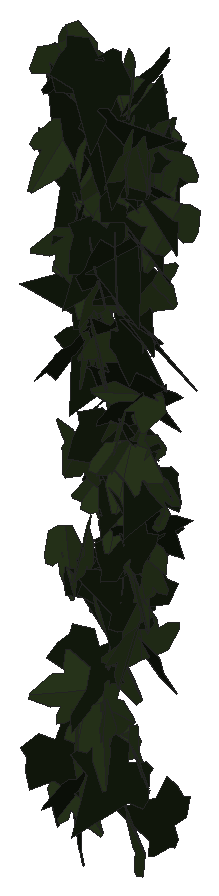
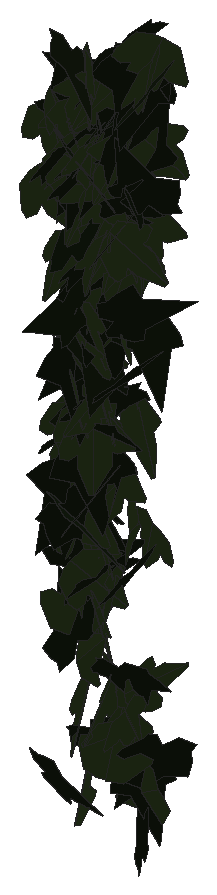
# SketchUp Ruby script. Lengths in inches.
U = 1.inch
M = Sketchup.active_model
def pt(a) = Geom::Point3d.new(a.map { |v| v * U })
def face(e, loops, mat)
  f = e.add_face(loops[0].map { |a| pt(a) })
  loops[1..].each { |l| e.add_face(l.map { |a| pt(a) }).erase! }
  f.material = f.back_material = mat if mat
  f
end
# faces: each face lists its corners as indices into pts; further lists are holes
def faces(e, pts, list, mat = nil) = list.each { |f| face(e, (f[0].is_a?(Array) ? f : [f]).map { |l| l.map { |i| pts[i] } }, mat) }
# xy, xz, yz: faces in a plane at the given z, y or x. An outline is a flat list of corners, or four numbers for a rectangle; further outlines are holes
def ring(l) = l.size == 4 ? [[l[0], l[1]], [l[2], l[1]], [l[2], l[3]], [l[0], l[3]]] : l.each_slice(2).to_a
def flat(e, list, mat, &to3) = list.each { |f| face(e, (f[0].is_a?(Array) ? f : [f]).map { |l| ring(l).map { |u, v| to3.(u, v) } }, mat) }
def xy(e, z, list, mat = nil) = flat(e, list, mat) { |x, y| [x, y, z] }
def xz(e, y, list, mat = nil) = flat(e, list, mat) { |x, z| [x, y, z] }
def yz(e, x, list, mat = nil) = flat(e, list, mat) { |y, z| [x, y, z] }
def lines(e, pts, list) = list.each { |a, b| e.add_line(pt(pts[a]), pt(pts[b])) }
# prism: a flat outline (further loops are holes) pulled along v
def prism(e, loops, v, mat = nil)
  f = face(e, loops, mat); d = Geom::Vector3d.new(v.map { |x| x * U })
  f.pushpull(f.normal.samedirection?(d) ? d.length : -d.length)
end
def box(e, o, s, mat = nil) = prism(e, [[o, [o[0] + s[0], o[1], o[2]], [o[0] + s[0], o[1] + s[1], o[2]], [o[0], o[1] + s[1], o[2]]]], [0, 0, s[2]], mat)
def at(x, y, z, deg = 0) = Geom::Transformation.translation(pt([x, y, z])) * Geom::Transformation.rotation(ORIGIN, Z_AXIS, deg.degrees)
def axes(o, x, y, z) = Geom::Transformation.new([*x, 0, *y, 0, *z, 0, *pt(o).to_a, 1])
def part(name) = M.definitions.add(name)
# library, detail: a bought-in or finely detailed component or shape, given as its bounding box
def library(name, o, s) = part(name).tap { |d| box(d.entities, o, s) }
def detail(e, o, s) = box(e.add_group.entities, o, s)
def put(e, d, t, mat = nil) = e.add_instance(d, t).tap { |i| i.material = mat if mat }
def group(e, t, mat = nil) = e.add_group.tap { |g| g.transformation = t; g.material = mat if mat }.entities
root = M.entities
M.materials.add("efeu1").color = [18, 25, 13]
M.materials.add("efeu2").color = [43, 57, 29]
c1 = part("ivyleaf_9")
p = [[1.54,2.16,1.25],[1.36,2.04,1.19],[-0.21,0.99,0.68],[-0.71,1.11,0.82],[-0.85,0.86,0.67],[-0.8,0.17,0.21],
  [-0.9,-0.01,0.1],[-0.67,-0.16,-0.02],[-0.08,-0.08,-0.05],[-0.03,-0.6,-0.4],[0.65,-0.88,-0.66],[0.83,-0.6,-0.49],
  [1.29,-0.42,-0.43],[1.8125,-0.07,-0.26],[1.21,0.44,0.15]]
faces(c1.entities,p,[[0,1,2,3,4,5,6,7,8,9,10,11,12,13,14]],"efeu1")
c2 = part("ivyleaf_10")
p = [[0,0.5,-0.03],[-0.0625,2.02,-0.43],[-0.19,2.01,-0.46],[-0.54,1.05,-0.29],[-0.52,0.625,-0.18],[-0.83,0.76,-0.28],
  [-1.16,0.64,-0.33],[-1.15,0.33,-0.24],[-0.77,-0.39,0.02],[-0.3,-0.51,0.16],[0.04,-0.48,0.23],[-0.02,2.01,-0.4375],
  [-0.06,2.01,-0.43],[0.04,-0.49,0.23],[0.67,-0.49,0.14],[1.38,0.36,-0.2],[1.375,0.51,-0.24],[0.81,0.65,-0.19],
  [0.62,0.59,-0.15],[0.6,1.09,-0.28],[0.5,1.23,-0.31]]
faces(c2.entities,p,[[0,1,2,3,4,5,6,7,8,9,10],[11,12,0,13,14,15,16,17,18,19,20]],"efeu2")
put(root,c1,axes([505.9,134.97,202.1],[-0.48741,0.05038,0.54087],[0.53842,-0.16422,0.46647],[0.16894,0.66872,0.0738]))
put(root,c2,axes([506.2,134.38,203.4],[0.33617,0.52917,-0.48557],[-0.31185,-0.37012,-0.63647],[-0.69544,0.42176,0.05069]))
put(root,c2,axes([505.99,134.85,205.88],[-0.15088,0.81193,-0.1575],[0.02758,-0.15507,-0.82583],[-0.82661,-0.15338,0.00119]))
put(root,c1,axes([506.57,135.38,198.56],[-0.26804,-0.09847,0.66727],[-0.6448,-0.23495,-0.27769],[0.27513,-0.64656,-0.00072]))
put(root,c1,axes([505.92,134.4,185.77],[-0.02694,-0.41849,-0.61943],[0.0465,0.59407,-0.43597],[0.78479,-0.04957,0.00457]))
put(root,c1,axes([505.94,135.15,183.02],[0.03534,-0.05301,0.72791],[0.1299,-0.68989,-0.06019],[0.74686,0.1225,-0.02398]))
put(root,c2,axes([506.81,134.96,200.54],[-0.36293,-0.14169,0.65201],[-0.60869,-0.27512,-0.37885],[0.33369,-0.65595,0.01806]))
put(root,c2,axes([506.47,134.6,187.4],[-0.10798,0.2032,0.71797],[-0.06576,-0.69688,0.20416],[0.77443,-0.03084,0.11744]))
put(root,c1,axes([505.91,134.95,205.33],[0.46062,-0.69476,-0.084],[0.0295,0.11975,-0.82867],[0.6992,0.45264,0.0903]))
put(root,c2,axes([506.36,135.26,186.92],[0.0782,0.58891,-0.37757],[-0.09629,-0.35405,-0.61577],[-0.74094,0.10817,0.04017]))
put(root,c2,axes([506.34,134.14,205.99],[-0.6972,-0.29211,-0.29478],[0.28746,0.09911,-0.73668],[0.33257,-0.69804,0.01877]))
put(root,c1,axes([506.6875,134.23,185],[-0.10898,0.67608,-0.20617],[0.0546,-0.1928,-0.71058],[-0.75894,-0.11095,-0.02152]))
put(root,c1,axes([506.54,135.14,202.08],[-0.43183,-0.55961,0.15094],[-0.09356,-0.11648,-0.71528],[0.61732,-0.40911,-0.00282]))
put(root,c1,axes([506.75,134.56,203.08],[0.50705,-0.04173,0.6532],[-0.6402,0.23427,0.47702],[-0.22869,-0.74835,0.11291]))
put(root,c1,axes([506.52,135.29,188.28],[-0.62142,-0.36737,-0.26252],[0.27785,0.06288,-0.70506],[0.39311,-0.62517,0.08335]))
put(root,c1,axes([506.85,133.81,197.85],[-0.14356,0.79952,-0.03224],[0.00115,-0.03125,-0.84291],[-0.86413,-0.13287,0.00423]))
put(root,c1,axes([506.61,134.27,205.44],[0.38487,0.63053,-0.04593],[-0.0249,-0.0377,-0.75323],[-0.68218,0.3571,0.00158]))
put(root,c1,axes([506.45,135.54,196.82],[-0.23751,-0.66097,0.36817],[0.03415,-0.39486,-0.68685],[0.75582,-0.18986,0.14672]))
put(root,c2,axes([506.74,134.18,200.81],[-0.5053,-0.64853,-0.00396],[0.00139,0.00376,-0.83167],[0.70043,-0.46787,-0.0012]))
put(root,c2,axes([506.03,134.62,184.59],[0.3965,-0.01317,0.74077],[0.74088,0.00762,-0.39643],[-0.00051,0.84017,0.01521]))
put(root,c2,axes([507.08,133.88,194.84],[-0.59609,0.10057,0.49608],[-0.50667,0.08625,-0.58346],[-0.14308,-0.72438,-0.0006]))
put(root,c2,axes([506.35,134.14,191.88],[0.63807,-0.18963,0.34261],[0.35843,-0.0395,-0.64265],[0.20015,0.67529,0.05862]))
put(root,c2,axes([506.85,135.38,185.4],[-0.62781,-0.39783,-0.1863],[-0.15963,-0.09612,0.74323],[-0.40925,0.64777,-0.00412]))
put(root,c2,axes([506.74,135.08,186.35],[0.49996,0.50856,-0.14226],[-0.09978,-0.10088,-0.71521],[-0.55995,0.47206,0.00042]))
put(root,c1,axes([506.64,135.43,203.98],[-0.05797,0.05272,-0.73545],[0.56163,-0.47922,-0.0782],[-0.52067,-0.52279,-0.00247]))
put(root,c1,axes([506.61,134.42,201.55],[-0.08415,0.57535,0.55617],[0.04479,-0.53364,0.60338],[0.84716,0.08536,0.02334]))
put(root,c1,axes([506.54,134.9,190.93],[0.28868,-0.7047,-0.12037],[-0.03109,0.11731,-0.76138],[0.71423,0.28994,0.01551]))
put(root,c1,axes([506.56,135.25,201.17],[0.39928,-0.70619,-0.07102],[-0.01722,0.07183,-0.811],[0.70954,0.39914,0.02029]))
put(root,c2,axes([506.85,134.5,191.96],[-0.07688,0.20886,-0.70763],[0.12741,-0.67089,-0.22701],[-0.75806,-0.13394,0.03361]))
put(root,c2,axes([506.93,134.47,200.11],[0.8266,0.09302,0.0051],[0.00501,0.00248,-0.80184],[-0.10048,0.76538,0.00198]))
put(root,c2,axes([506.86,134.67,198.08],[0.28754,-0.5142,0.53683],[0.34895,-0.40924,-0.5973],[0.70527,0.41212,0.07667]))
put(root,c2,axes([506.96,134.61,203.16],[0.11167,0.65461,0.43041],[0.02152,0.41514,-0.68808],[-0.83614,0.09811,0.03977]))
put(root,c2,axes([507.21,134.53,190.43],[-0.2462,0.47178,0.4209],[-0.20846,0.35603,-0.54471],[-0.63813,-0.29833,0.01555]))
put(root,c2,axes([507.23,134.26,199.54],[-0.7868,0.29407,-0.09976],[0.09346,-0.04187,-0.81703],[-0.32072,-0.73361,0.00664]))
put(root,c2,axes([507.66,135.45,190.82],[-0.3494,-0.35385,0.57863],[-0.29236,-0.49382,-0.49033],[0.64933,-0.41274,0.09058]))
put(root,c2,axes([507.41,134.65,193.42],[-0.78212,-0.20437,-0.07107],[0.06891,0.02548,-0.78253],[0.22229,-0.72696,-0.00745]))
put(root,c2,axes([507.39,134.62,187.12],[0.22352,-0.47181,-0.62714],[0.06767,0.66124,-0.47335],[0.78188,0.07766,0.22025]))
put(root,c2,axes([507.2,134.45,200.51],[0.3411,0.60844,0.42613],[0.1273,0.41409,-0.69315],[-0.73183,0.35562,0.07804]))
put(root,c1,axes([507.23,134.39,205.99],[-0.07291,-0.83658,0.02971],[0.00071,-0.02989,-0.83975],[0.83711,-0.07284,0.0033]))
put(root,c2,axes([507.93,135.03,192.15],[-0.57202,0.2865,-0.47924],[-0.4593,0.18076,0.62523],[0.36396,0.67838,0.0358]))
put(root,c2,axes([507.49,135.11,189.86],[0.60838,-0.5967,0.00898],[0.00677,-0.00591,-0.85216],[0.59673,0.60842,0.00052]))
put(root,c1,axes([507.7,134.875,194.05],[0.34677,0.50768,-0.38385],[-0.20514,-0.31654,-0.62468],[-0.64609,0.37299,-0.00768]))
put(root,c2,axes([507.66,135.03,194.66],[-0.54907,-0.5484,0.00044],[0.00538,-0.00519,-0.77768],[0.59224,-0.50837,0.00747]))
put(root,c1,axes([507.37,135.2,190.65],[-0.08634,-0.75429,-0.01122],[-0.00292,0.01162,-0.7592],[0.75437,-0.08629,-0.00422]))
put(root,c1,axes([507.8,134.54,200.9],[-0.74349,-0.30747,0.00273],[-0.00234,-0.00158,-0.78412],[0.33208,-0.68842,0.00058]))
put(root,c2,axes([507.52,134.96,200.24],[-0.14291,0.68465,0.09871],[-0.034,0.09057,-0.72507],[-0.74572,-0.13533,0.01414]))
put(root,c2,axes([507.12,134.32,198.13],[0.29318,-0.3648,0.60841],[0.61302,-0.2386,-0.42867],[0.42263,0.59916,0.19972]))
put(root,c2,axes([507.99,134.8125,201.24],[0.16644,0.31389,0.63151],[-0.49349,-0.41564,0.34406],[0.54905,-0.46873,0.11781]))
put(root,c2,axes([507.49,134,200.86],[-0.28951,0.64386,-0.16028],[0.0694,-0.14018,-0.72531],[-0.71164,-0.27561,-0.00553]))
put(root,c1,axes([507.82,134.39,196.67],[0.08879,0.62516,0.36414],[-0.07213,0.35759,-0.64769],[-0.77049,0.03856,0.1026]))
put(root,c2,axes([507.48,134.0625,202.32],[0.06736,-0.29867,0.68359],[0.06153,0.65973,0.30615],[-0.7773,0.02634,0.08348]))
put(root,c2,axes([507.61,135.16,203.12],[0.07754,0.66937,-0.09632],[-0.02797,-0.09034,-0.69994],[-0.72927,0.07464,0.0166]))
put(root,c2,axes([508.07,134.82,187.9],[-0.39226,0.30403,-0.44186],[-0.36805,0.25434,0.49226],[0.42767,0.49773,0.01835]))
put(root,c2,axes([507.78,133.73,199.93],[-0.00169,-0.56015,-0.53529],[0.02763,0.51437,-0.58226],[0.8211,-0.01846,0.0185]))
put(root,c2,axes([507.67,134.63,195.62],[-0.09451,-0.27106,-0.735],[0.18417,0.68609,-0.29563],[0.79647,-0.19081,-0.01886]))
put(root,c2,axes([507.83,134.49,195.88],[0.50129,-0.58628,-0.21726],[-0.13097,0.17042,-0.77761],[0.65929,0.47963,0.01072]))
put(root,c2,axes([507.54,134.2,201.5],[-0.2278,-0.30885,-0.61673],[0.38163,0.4764,-0.38876],[0.61303,-0.41134,0.01283]))
put(root,c2,axes([507.49,134.95,191.48],[0.52123,-0.36531,0.33957],[0.31481,-0.15431,-0.62764],[0.42533,0.56189,0.04841]))
put(root,c1,axes([507.94,134.64,185.73],[-0.66676,-0.40237,0.01917],[-0.01624,-0.01018,-0.77877],[0.4025,-0.66696,0.00032]))
put(root,c2,axes([507.64,134.97,201.73],[-0.71869,-0.24262,-0.27889],[0.28265,0.06446,-0.7361],[0.26953,-0.71456,0.02829]))
put(root,c2,axes([507.76,134.95,191.85],[0.72959,-0.17745,-0.13262],[-0.08391,0.20108,-0.73069],[0.20502,0.71377,0.17287]))
put(root,c2,axes([507.79,134.34,198.17],[-0.41122,-0.54336,-0.1912],[0.1156,0.14949,-0.69003],[0.60863,-0.39552,0.00188]))
put(root,c2,axes([507.38,134.25,186.98],[0.65246,-0.25281,0.5036],[0.47256,-0.17419,-0.69969],[0.30694,0.80558,0.00674]))
put(root,c1,axes([508.375,134.98,192.12],[-0.45582,0.53306,0.31299],[-0.32523,0.13746,-0.69242],[-0.57559,-0.49981,0.14338]))
put(root,c2,axes([507.79,135.04,205.5],[0.52207,-0.6319,-0.15656],[0.03436,0.22715,-0.80224],[0.6501,0.49545,0.16813]))
put(root,c2,axes([508.02,134.86,198],[0.51558,-0.35857,-0.36785],[-0.30687,0.21066,-0.62093],[0.44914,0.55555,-0.00197]))
put(root,c1,axes([507.8125,134.26,198.52],[0.54701,0.42102,-0.21384],[-0.169,-0.13342,-0.68497],[-0.47698,0.53011,-0.00255]))
put(root,c1,axes([507.49,135.32,192.89],[0.20655,-0.75847,0.16522],[0.03911,-0.16058,-0.78608],[0.77527,0.21018,-0.00436]))
put(root,c1,axes([507.91,134.86,194.57],[-0.64244,-0.39994,-0.2115],[0.18233,0.11337,-0.74547],[0.44896,-0.61835,0.00012]))
put(root,c1,axes([508.15,135.4,192.55],[0.01162,0.16304,-0.67841],[-0.11569,-0.64365,-0.16915],[-0.7169,0.10652,0.0163]))
put(root,c1,axes([507.65,134.02,203.79],[0.50127,-0.44874,-0.41976],[-0.27302,0.31781,-0.6698],[0.59191,0.52662,0.04653]))
put(root,c2,axes([507.85,134.54,193.5625],[0.70397,0.3595,-0.09635],[-0.09813,-0.02701,-0.77389],[-0.38875,0.65782,0.02087]))
put(root,c1,axes([508.41,134.96,202.72],[-0.46894,0.44729,0.27331],[-0.20799,0.17923,-0.64819],[-0.52024,-0.47484,0.01279]))
put(root,c2,axes([507.79,134.52,200.68],[-0.22018,0.53236,-0.40274],[0.10654,-0.37611,-0.59174],[-0.70294,-0.22375,0.03646]))
put(root,c2,axes([507.99,134.7,201.125],[-0.01278,-0.2543,-0.6565],[0.02216,0.63092,-0.26474],[0.73466,-0.02345,-0.00344]))
put(root,c1,axes([507.67,134.58,195.45],[-0.10009,-0.79739,-0.26224],[0.09332,0.25189,-0.80153],[0.8342,-0.12385,0.0582]))
put(root,c1,axes([508.47,134.85,190.46],[-0.12991,0.028,0.74052],[-0.76459,-0.08688,-0.12083],[0.08759,-0.71688,0.04357]))
put(root,c2,axes([507.55,134.64,204.45],[0.5058,0.31332,0.47004],[0.39415,0.26701,-0.58581],[-0.4443,0.59355,0.01541]))
put(root,c2,axes([507.77,134.92,204.88],[0.29609,0.58755,0.23519],[0.0957,0.20818,-0.67426],[-0.67316,0.28803,0.00759]))
put(root,c1,axes([507.67,134.83,199.95],[0.22362,-0.74609,-0.22897],[0.00382,0.23923,-0.77579],[0.78043,0.21261,0.06941]))
put(root,c1,axes([507.96,134.4,202.49],[0.5522,0.46195,-0.0992],[-0.08293,-0.05727,-0.71657],[-0.50263,0.51695,0.00925]))
put(root,c2,axes([508.52,134.84,193.95],[-0.42828,0.08465,-0.5291],[-0.54658,0.05966,0.42059],[0.10721,0.64228,0.03067]))
put(root,c2,axes([508.16,134.81,194.91],[-0.39841,-0.60019,-0.01875],[0.02019,0.00967,-0.73259],[0.64818,-0.36921,0.01129]))
put(root,c1,axes([507.7,135.14,203.35],[0.49721,-0.61826,-0.23493],[-0.0779,0.23712,-0.7889],[0.65679,0.49617,0.08428]))
put(root,c1,axes([508.48,134.84,205.52],[-0.23251,0.61055,0.25771],[-0.13142,0.21937,-0.67206],[-0.69939,-0.24419,0.04061]))
put(root,c1,axes([507.87,135.6,200.24],[0.61907,-0.42446,-0.1539],[0.12855,-0.08792,0.74179],[-0.46815,-0.58544,0.00018]))
put(root,c1,axes([507.83,135.04,202.38],[0.17543,-0.74114,-0.30585],[-0.03434,0.30586,-0.76084],[0.80103,0.17543,0.03437]))
put(root,c2,axes([507.86,134.99,197.09],[0.6837,-0.09079,0.26191],[0.27205,-0.01684,-0.66486],[0.09787,0.6811,0.01847]))
put(root,c1,axes([507.8,134.1,201.34],[0.08565,-0.79889,-0.33388],[0.05836,0.34007,-0.79874],[0.86389,0.05623,0.08706]))
put(root,c1,axes([507.93,134.52,204.45],[-0.01139,-0.817,0.15386],[-0.02829,-0.1534,-0.81668],[0.83088,-0.01642,-0.0257]))
put(root,c1,axes([507.93,133.62,200.15],[0.06818,-0.04116,0.79745],[0.58042,0.55189,-0.0152],[-0.59234,0.53604,0.07689]))
put(root,c2,axes([508.25,134.36,195.125],[0.04119,-0.78152,0.03553],[0.00369,-0.03403,-0.81375],[0.84484,0.03825,0.00182]))
put(root,c2,axes([508.75,134.49,196.78],[0.17034,0.09038,-0.73299],[-0.7674,0.02335,-0.16226],[0.0035,0.72185,0.09703]))
put(root,c1,axes([508.34,134.49,196.42],[0.2215,0.7006,-0.12347],[-0.04803,-0.11067,-0.75911],[-0.76593,0.20955,0.01189]))
put(root,c2,axes([508.68,134.72,193.67],[-0.48424,0.00062,0.55348],[-0.55873,-0.16373,-0.4531],[0.13481,-0.67635,0.1102]))
put(root,c1,axes([508.51,133.97,192.11],[-0.71334,0.33229,-0.04809],[-0.04799,0.01457,0.76892],[0.35914,0.66196,0.00722]))
put(root,c2,axes([508.5,135.11,202.69],[0.33439,0.33639,-0.51279],[-0.44049,-0.28632,-0.46951],[-0.47067,0.50695,0.07509]))
put(root,c2,axes([508.77,133.66,203.83],[-0.01924,0.16408,0.83402],[-0.72198,0.43714,-0.10265],[-0.44862,-0.71054,0.12944]))
put(root,c2,axes([508.2,134.73,194.91],[0.56404,-0.48645,0.08064],[-0.04252,0.07142,0.7418],[-0.5303,-0.52313,0.02628]))
put(root,c2,axes([508.29,134.91,189.07],[-0.37449,-0.75009,-0.1809],[-0.0483,-0.17789,0.83762],[-0.77008,0.37592,0.03543]))
put(root,c2,axes([508.22,134.79,183.37],[-0.56539,0.47625,0.41907],[0.28992,-0.30531,0.73812],[0.56425,0.63409,0.04065]))
put(root,c1,axes([507.98,134.09,197.28],[0.85412,0.19363,0.00813],[0.00719,0.00506,-0.87579],[-0.19366,0.85415,0.00335]))
put(root,c2,axes([508.39,134.3,189.71],[0.16483,-0.73635,0.01947],[-0.00472,-0.021,-0.75452],[0.73659,0.16464,-0.00919]))
put(root,c2,axes([508.48,134.39,186.44],[-0.52422,0.51043,0.28692],[-0.20068,0.20516,-0.73164],[-0.55008,-0.56128,-0.00651]))
put(root,c1,axes([507.74,134.05,204.2],[0.5431,0.21367,-0.50358],[0.4392,0.27149,0.56382],[0.36583,-0.64314,0.07071]))
put(root,c2,axes([508.34,134.99,204.1],[0.23921,0.64445,-0.0855],[-0.04114,-0.07382,-0.7086],[-0.70044,0.22443,0.01242]))
put(root,c1,axes([507.95,134.98,195.2],[0.43053,-0.5168,0.23622],[0.16591,-0.16825,-0.67854],[0.58667,0.42684,0.01854]))
put(root,c1,axes([507.94,135.35,188.75],[0.65068,-0.18816,-0.40424],[0.40429,-0.05265,0.67526],[-0.18806,-0.76421,0.05301]))
put(root,c2,axes([508.43,134.07,195.04],[0.70358,0.27743,-0.07825],[-0.07538,-0.02813,-0.7364],[-0.30115,0.65519,0.00151]))
put(root,c2,axes([508.77,134.34,191.91],[-0.66198,0.04801,0.23019],[-0.23998,-0.0039,-0.63908],[-0.04734,-0.65167,0.02078]))
put(root,c1,axes([508.41,134.54,192.84],[0.52323,0.56044,0.06902],[0.05125,0.04657,-0.7667],[-0.56235,0.5257,-0.00566]))
put(root,c1,axes([509.09,135.07,184.23],[-0.44134,0.28396,0.46049],[-0.39026,0.2559,-0.51751],[-0.41282,-0.54549,-0.00307]))
put(root,c1,axes([508.51,134.57,203.62],[-0.58211,-0.1002,0.4736],[0.49268,0.03068,0.56856],[-0.10418,0.70494,0.04258]))
put(root,c1,axes([508.38,133.92,198.67],[0.52028,-0.29816,-0.4886],[-0.34983,0.35499,-0.57974],[0.48862,0.57164,0.10518]))
put(root,c2,axes([508.49,134.47,191.45],[-0.28126,0.62793,-0.10896],[0.04637,-0.09562,-0.70698],[-0.68598,-0.26392,-0.00312]))
put(root,c1,axes([508.1,135.08,198.24],[0.62776,-0.31892,0.16725],[0.149,-0.08286,-0.68949],[0.3558,0.59738,-0.00635]))
put(root,c1,axes([508.31,135.28,202.99],[0.19861,-0.7746,-0.18675],[-0.04181,0.18207,-0.79965],[0.7957,0.20291,0.0046]))
put(root,c2,axes([508.58,135.02,191.375],[-0.11888,0.38106,0.62309],[0.1864,-0.57374,0.41249],[0.74384,0.20467,-0.00378]))
put(root,c2,axes([508.6875,134.9,199.74],[-0.13732,-0.52073,-0.45253],[0.09276,0.42679,-0.55729],[0.72699,-0.15281,-0.01437]))
put(root,c1,axes([508.6,134.97,194.36],[-0.24922,-0.68277,0.30544],[0.04532,-0.33514,-0.71219],[0.7466,-0.20758,0.14519]))
put(root,c2,axes([508.8,135.11,204.17],[0.08172,-0.66024,0.18762],[0.05459,-0.17562,-0.69048],[0.73718,0.0862,0.03033]))
put(root,c2,axes([508.91,134.43,194.44],[-0.75444,0.08237,0.07675],[-0.07943,0.00645,-0.73152],[-0.0892,-0.70241,0.00228]))
put(root,c2,axes([508.85,134,204.05],[-0.16827,-0.75005,-0.31521],[0.06886,0.3076,-0.76869],[0.81067,-0.18182,-0.00013]))
put(root,c2,axes([508.41,134.9375,203.68],[0.19108,-0.16328,0.68654],[0.55741,-0.4119,-0.24982],[0.47821,0.54536,0.01687]))
put(root,c2,axes([509.04,134.97,203.55],[-0.68389,-0.22488,0.1822],[-0.17523,-0.06659,-0.69881],[0.25314,-0.65364,0.00851]))
put(root,c2,axes([509.05,135.2,201.78],[-0.38928,-0.61442,0.38107],[-0.08552,-0.39063,-0.71719],[0.71793,-0.37969,0.1212]))
